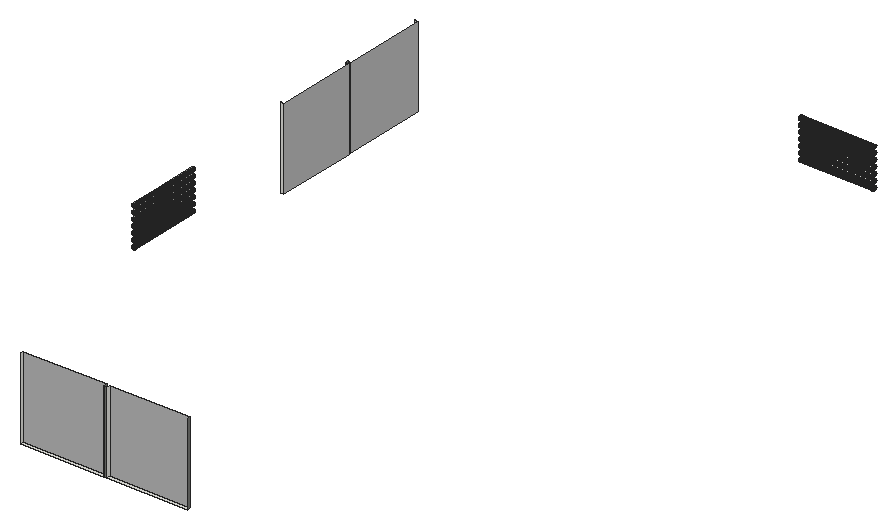
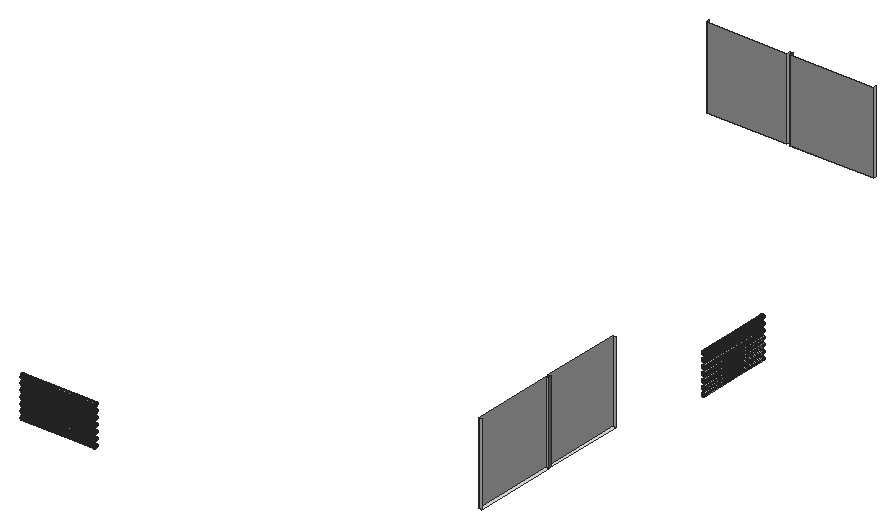
# SketchUp Ruby script. Lengths in inches.
U = 1.inch
M = Sketchup.active_model
def pt(a) = Geom::Point3d.new(a.map { |v| v * U })
def face(e, loops, mat)
  f = e.add_face(loops[0].map { |a| pt(a) })
  loops[1..].each { |l| e.add_face(l.map { |a| pt(a) }).erase! }
  f.material = f.back_material = mat if mat
  f
end
# faces: each face lists its corners as indices into pts; further lists are holes
def faces(e, pts, list, mat = nil) = list.each { |f| face(e, (f[0].is_a?(Array) ? f : [f]).map { |l| l.map { |i| pts[i] } }, mat) }
# xy, xz, yz: faces in a plane at the given z, y or x. An outline is a flat list of corners, or four numbers for a rectangle; further outlines are holes
def ring(l) = l.size == 4 ? [[l[0], l[1]], [l[2], l[1]], [l[2], l[3]], [l[0], l[3]]] : l.each_slice(2).to_a
def flat(e, list, mat, &to3) = list.each { |f| face(e, (f[0].is_a?(Array) ? f : [f]).map { |l| ring(l).map { |u, v| to3.(u, v) } }, mat) }
def xy(e, z, list, mat = nil) = flat(e, list, mat) { |x, y| [x, y, z] }
def xz(e, y, list, mat = nil) = flat(e, list, mat) { |x, z| [x, y, z] }
def yz(e, x, list, mat = nil) = flat(e, list, mat) { |y, z| [x, y, z] }
def lines(e, pts, list) = list.each { |a, b| e.add_line(pt(pts[a]), pt(pts[b])) }
# prism: a flat outline (further loops are holes) pulled along v
def prism(e, loops, v, mat = nil)
  f = face(e, loops, mat); d = Geom::Vector3d.new(v.map { |x| x * U })
  f.pushpull(f.normal.samedirection?(d) ? d.length : -d.length)
end
def box(e, o, s, mat = nil) = prism(e, [[o, [o[0] + s[0], o[1], o[2]], [o[0] + s[0], o[1] + s[1], o[2]], [o[0], o[1] + s[1], o[2]]]], [0, 0, s[2]], mat)
def at(x, y, z, deg = 0) = Geom::Transformation.translation(pt([x, y, z])) * Geom::Transformation.rotation(ORIGIN, Z_AXIS, deg.degrees)
def axes(o, x, y, z) = Geom::Transformation.new([*x, 0, *y, 0, *z, 0, *pt(o).to_a, 1])
def part(name) = M.definitions.add(name)
# library, detail: a bought-in or finely detailed component or shape, given as its bounding box
def library(name, o, s) = part(name).tap { |d| box(d.entities, o, s) }
def detail(e, o, s) = box(e.add_group.entities, o, s)
def put(e, d, t, mat = nil) = e.add_instance(d, t).tap { |i| i.material = mat if mat }
def group(e, t, mat = nil) = e.add_group.tap { |g| g.transformation = t; g.material = mat if mat }.entities
root = M.entities
M.materials.add("[Metal Seamed]").color = [118, 119, 115]
M.materials.add("[Mirror 01]").color = [185, 185, 185]
xy(root,539.76,[[312.65,102.8125,473.9375,108.8125],[479.9375,102.8125,635.22,108.8125],[138,949.59,144,1104.875],[138,1110.875,144,1272.16]])
xz(root,102.8125,[[473.9375,539.76,479.9375,696.625]],"[Metal Seamed]")
xz(root,108.8125,[[312.65,539.76,473.9375,696.625],[479.9375,539.76,635.22,696.625]],"[Mirror 01]")
xz(root,949.59,[[138,539.76,144,696.625]])
xz(root,1104.875,[[138,539.76,144,696.625]])
xz(root,1110.875,[[138,539.76,144,696.625]])
xz(root,1272.16,[[138,539.76,144,696.625]])
yz(root,138,[[1104.875,539.76,1110.875,696.625]],"[Metal Seamed]")
yz(root,144,[[949.59,539.76,1104.875,696.625],[1110.875,539.76,1272.16,696.625]],"[Mirror 01]")
yz(root,312.65,[[102.8125,539.76,108.8125,696.625]])
yz(root,473.9375,[[102.8125,539.76,108.8125,696.625]],"[Metal Seamed]")
yz(root,479.9375,[[102.8125,539.76,108.8125,696.625]])
yz(root,635.22,[[102.8125,539.76,108.8125,696.625]],"[Metal Seamed]")
p = [[83.53,662.8,549.02],[82.57,662.8,549.14],[82.57,806.17,549.14],[83.53,806.17,549.02],[84.48,662.8,549.14],[84.48,806.17,549.14],
  [697.99,1500.33,549.14],[697.99,1501.28,549.02],[841.36,1501.28,549.02],[841.36,1500.33,549.14],[697.99,1502.24,549.14],[841.36,1502.24,549.14],
  [81.68,662.8,549.51],[81.68,806.17,549.51],[85.37,662.8,549.51],[85.37,806.17,549.51],[697.99,1499.44,549.51],[841.36,1499.44,549.51],
  [697.99,1503.13,549.51],[841.36,1503.13,549.51],[80.92,662.8,550.1],[80.92,806.17,550.1],[86.13,662.8,550.1],[86.13,806.17,550.1],
  [697.99,1498.68,550.1],[841.36,1498.68,550.1],[697.99,1503.89,550.1],[841.36,1503.89,550.1],[80.33,662.8,550.86],[80.33,806.17,550.86],
  [86.72,662.8,550.86],[86.72,806.17,550.86],[697.99,1498.09,550.86],[841.36,1498.09,550.86],[697.99,1504.48,550.86],[841.36,1504.48,550.86],
  [79.97,662.8,551.75],[79.97,806.17,551.75],[87.09,662.8,551.75],[87.09,806.17,551.75],[697.99,1497.72,551.75],[841.36,1497.72,551.75],
  [697.99,1504.85,551.75],[841.36,1504.85,551.75],[79.84,662.8,552.7],[79.84,806.17,552.7],[87.21,662.8,552.7],[87.21,806.17,552.7],
  [697.99,1497.6,552.7],[841.36,1497.6,552.7],[697.99,1504.97,552.7],[841.36,1504.97,552.7],[79.97,662.8,553.66],[79.97,806.17,553.66],
  [87.09,662.8,553.66],[87.09,806.17,553.66],[697.99,1497.72,553.66],[841.36,1497.72,553.66],[697.99,1504.85,553.66],[841.36,1504.85,553.66],
  [80.33,662.8,554.55],[80.33,806.17,554.55],[86.72,662.8,554.55],[86.72,806.17,554.55],[697.99,1498.09,554.55],[841.36,1498.09,554.55],
  [697.99,1504.48,554.55],[841.36,1504.48,554.55],[80.92,662.8,555.3125],[80.92,806.17,555.3125],[86.13,662.8,555.3125],[86.13,806.17,555.3125],
  [697.99,1498.68,555.3125],[841.36,1498.68,555.3125],[697.99,1503.89,555.3125],[841.36,1503.89,555.3125],[81.68,662.8,555.9],[81.68,806.17,555.9],
  [85.37,662.8,555.9],[85.37,806.17,555.9],[697.99,1499.44,555.9],[841.36,1499.44,555.9],[697.99,1503.13,555.9],[841.36,1503.13,555.9],
  [82.57,662.8,556.27],[82.57,806.17,556.27],[84.48,662.8,556.27],[84.48,806.17,556.27],[697.99,1500.33,556.27],[841.36,1500.33,556.27],
  [697.99,1502.24,556.27],[841.36,1502.24,556.27],[83.53,662.8,556.39],[83.53,806.17,556.39],[697.99,1501.28,556.39],[841.36,1501.28,556.39],
  [83.53,662.8,561.02],[82.57,662.8,561.14],[82.57,806.17,561.14],[83.53,806.17,561.02],[84.48,662.8,561.14],[84.48,806.17,561.14],
  [697.99,1500.33,561.14],[697.99,1501.28,561.02],[841.36,1501.28,561.02],[841.36,1500.33,561.14],[697.99,1502.24,561.14],[841.36,1502.24,561.14],
  [81.68,662.8,561.51],[81.68,806.17,561.51],[85.37,662.8,561.51],[85.37,806.17,561.51],[697.99,1499.44,561.51],[841.36,1499.44,561.51],
  [697.99,1503.13,561.51],[841.36,1503.13,561.51],[80.92,662.8,562.1],[80.92,806.17,562.1],[86.13,662.8,562.1],[86.13,806.17,562.1],
  [697.99,1498.68,562.1],[841.36,1498.68,562.1],[697.99,1503.89,562.1],[841.36,1503.89,562.1],[80.33,662.8,562.86],[80.33,806.17,562.86],
  [86.72,662.8,562.86],[86.72,806.17,562.86],[697.99,1498.09,562.86],[841.36,1498.09,562.86],[697.99,1504.48,562.86],[841.36,1504.48,562.86],
  [79.97,662.8,563.75],[79.97,806.17,563.75],[87.09,662.8,563.75],[87.09,806.17,563.75],[697.99,1497.72,563.75],[841.36,1497.72,563.75],
  [697.99,1504.85,563.75],[841.36,1504.85,563.75],[79.84,662.8,564.7],[79.84,806.17,564.7],[87.21,662.8,564.7],[87.21,806.17,564.7],
  [697.99,1497.6,564.7],[841.36,1497.6,564.7],[697.99,1504.97,564.7],[841.36,1504.97,564.7],[79.97,662.8,565.66],[79.97,806.17,565.66],
  [87.09,662.8,565.66],[87.09,806.17,565.66],[697.99,1497.72,565.66],[841.36,1497.72,565.66],[697.99,1504.85,565.66],[841.36,1504.85,565.66],
  [80.33,662.8,566.55],[80.33,806.17,566.55],[86.72,662.8,566.55],[86.72,806.17,566.55],[697.99,1498.09,566.55],[841.36,1498.09,566.55],
  [697.99,1504.48,566.55],[841.36,1504.48,566.55],[80.92,662.8,567.3125],[80.92,806.17,567.3125],[86.13,662.8,567.3125],[86.13,806.17,567.3125],
  [697.99,1498.68,567.3125],[841.36,1498.68,567.3125],[697.99,1503.89,567.3125],[841.36,1503.89,567.3125],[81.68,662.8,567.9],[81.68,806.17,567.9],
  [85.37,662.8,567.9],[85.37,806.17,567.9],[697.99,1499.44,567.9],[841.36,1499.44,567.9],[697.99,1503.13,567.9],[841.36,1503.13,567.9],
  [82.57,662.8,568.27],[82.57,806.17,568.27],[84.48,662.8,568.27],[84.48,806.17,568.27],[697.99,1500.33,568.27],[841.36,1500.33,568.27],
  [697.99,1502.24,568.27],[841.36,1502.24,568.27],[83.53,662.8,568.39],[83.53,806.17,568.39],[697.99,1501.28,568.39],[841.36,1501.28,568.39],
  [83.53,662.8,573.02],[82.57,662.8,573.14],[82.57,806.17,573.14],[83.53,806.17,573.02],[84.48,662.8,573.14],[84.48,806.17,573.14],
  [697.99,1500.33,573.14],[697.99,1501.28,573.02],[841.36,1501.28,573.02],[841.36,1500.33,573.14],[697.99,1502.24,573.14],[841.36,1502.24,573.14],
  [81.68,662.8,573.51],[81.68,806.17,573.51],[85.37,662.8,573.51],[85.37,806.17,573.51],[697.99,1499.44,573.51],[841.36,1499.44,573.51],
  [697.99,1503.13,573.51],[841.36,1503.13,573.51],[80.92,662.8,574.1],[80.92,806.17,574.1],[86.13,662.8,574.1],[86.13,806.17,574.1],
  [697.99,1498.68,574.1],[841.36,1498.68,574.1],[697.99,1503.89,574.1],[841.36,1503.89,574.1],[80.33,662.8,574.86],[80.33,806.17,574.86],
  [86.72,662.8,574.86],[86.72,806.17,574.86],[697.99,1498.09,574.86],[841.36,1498.09,574.86],[697.99,1504.48,574.86],[841.36,1504.48,574.86],
  [79.97,662.8,575.75],[79.97,806.17,575.75],[87.09,662.8,575.75],[87.09,806.17,575.75],[697.99,1497.72,575.75],[841.36,1497.72,575.75],
  [697.99,1504.85,575.75],[841.36,1504.85,575.75],[79.84,662.8,576.7],[79.84,806.17,576.7],[87.21,662.8,576.7],[87.21,806.17,576.7],
  [697.99,1497.6,576.7],[841.36,1497.6,576.7],[697.99,1504.97,576.7],[841.36,1504.97,576.7],[79.97,662.8,577.66],[79.97,806.17,577.66],
  [87.09,662.8,577.66],[87.09,806.17,577.66],[697.99,1497.72,577.66],[841.36,1497.72,577.66],[697.99,1504.85,577.66],[841.36,1504.85,577.66],
  [80.33,662.8,578.55],[80.33,806.17,578.55],[86.72,662.8,578.55],[86.72,806.17,578.55],[697.99,1498.09,578.55],[841.36,1498.09,578.55],
  [697.99,1504.48,578.55],[841.36,1504.48,578.55],[80.92,662.8,579.3125],[80.92,806.17,579.3125],[86.13,662.8,579.3125],[86.13,806.17,579.3125],
  [697.99,1498.68,579.3125],[841.36,1498.68,579.3125],[697.99,1503.89,579.3125],[841.36,1503.89,579.3125],[81.68,662.8,579.9],[81.68,806.17,579.9],
  [85.37,662.8,579.9],[85.37,806.17,579.9],[697.99,1499.44,579.9],[841.36,1499.44,579.9],[697.99,1503.13,579.9],[841.36,1503.13,579.9],
  [82.57,662.8,580.27],[82.57,806.17,580.27],[84.48,662.8,580.27],[84.48,806.17,580.27],[697.99,1500.33,580.27],[841.36,1500.33,580.27],
  [697.99,1502.24,580.27],[841.36,1502.24,580.27],[83.53,662.8,580.39],[83.53,806.17,580.39],[697.99,1501.28,580.39],[841.36,1501.28,580.39],
  [83.53,662.8,585.02],[82.57,662.8,585.14],[82.57,806.17,585.14],[83.53,806.17,585.02],[84.48,662.8,585.14],[84.48,806.17,585.14],
  [697.99,1500.33,585.14],[697.99,1501.28,585.02],[841.36,1501.28,585.02],[841.36,1500.33,585.14],[697.99,1502.24,585.14],[841.36,1502.24,585.14],
  [81.68,662.8,585.51],[81.68,806.17,585.51],[85.37,662.8,585.51],[85.37,806.17,585.51],[697.99,1499.44,585.51],[841.36,1499.44,585.51],
  [697.99,1503.13,585.51],[841.36,1503.13,585.51],[80.92,662.8,586.1],[80.92,806.17,586.1],[86.13,662.8,586.1],[86.13,806.17,586.1],
  [697.99,1498.68,586.1],[841.36,1498.68,586.1],[697.99,1503.89,586.1],[841.36,1503.89,586.1],[80.33,662.8,586.86],[80.33,806.17,586.86],
  [86.72,662.8,586.86],[86.72,806.17,586.86],[697.99,1498.09,586.86],[841.36,1498.09,586.86],[697.99,1504.48,586.86],[841.36,1504.48,586.86],
  [79.97,662.8,587.75],[79.97,806.17,587.75],[87.09,662.8,587.75],[87.09,806.17,587.75],[697.99,1497.72,587.75],[841.36,1497.72,587.75],
  [697.99,1504.85,587.75],[841.36,1504.85,587.75],[79.84,662.8,588.7],[79.84,806.17,588.7],[87.21,662.8,588.7],[87.21,806.17,588.7],
  [697.99,1497.6,588.7],[841.36,1497.6,588.7],[697.99,1504.97,588.7],[841.36,1504.97,588.7],[79.97,662.8,589.66],[79.97,806.17,589.66],
  [87.09,662.8,589.66],[87.09,806.17,589.66],[697.99,1497.72,589.66],[841.36,1497.72,589.66],[697.99,1504.85,589.66],[841.36,1504.85,589.66],
  [80.33,662.8,590.55],[80.33,806.17,590.55],[86.72,662.8,590.55],[86.72,806.17,590.55],[697.99,1498.09,590.55],[841.36,1498.09,590.55],
  [697.99,1504.48,590.55],[841.36,1504.48,590.55],[80.92,662.8,591.3125],[80.92,806.17,591.3125],[86.13,662.8,591.3125],[86.13,806.17,591.3125],
  [697.99,1498.68,591.3125],[841.36,1498.68,591.3125],[697.99,1503.89,591.3125],[841.36,1503.89,591.3125],[81.68,662.8,591.9],[81.68,806.17,591.9],
  [85.37,662.8,591.9],[85.37,806.17,591.9],[697.99,1499.44,591.9],[841.36,1499.44,591.9],[697.99,1503.13,591.9],[841.36,1503.13,591.9],
  [82.57,662.8,592.27],[82.57,806.17,592.27],[84.48,662.8,592.27],[84.48,806.17,592.27],[697.99,1500.33,592.27],[841.36,1500.33,592.27],
  [697.99,1502.24,592.27],[841.36,1502.24,592.27],[83.53,662.8,592.39],[83.53,806.17,592.39],[697.99,1501.28,592.39],[841.36,1501.28,592.39],
  [83.53,662.8,597.02],[82.57,662.8,597.14],[82.57,806.17,597.14],[83.53,806.17,597.02],[84.48,662.8,597.14],[84.48,806.17,597.14],
  [697.99,1500.33,597.14],[697.99,1501.28,597.02],[841.36,1501.28,597.02],[841.36,1500.33,597.14],[697.99,1502.24,597.14],[841.36,1502.24,597.14],
  [81.68,662.8,597.51],[81.68,806.17,597.51],[85.37,662.8,597.51],[85.37,806.17,597.51],[697.99,1499.44,597.51],[841.36,1499.44,597.51],
  [697.99,1503.13,597.51],[841.36,1503.13,597.51],[80.92,662.8,598.1],[80.92,806.17,598.1],[86.13,662.8,598.1],[86.13,806.17,598.1],
  [697.99,1498.68,598.1],[841.36,1498.68,598.1],[697.99,1503.89,598.1],[841.36,1503.89,598.1],[80.33,662.8,598.86],[80.33,806.17,598.86],
  [86.72,662.8,598.86],[86.72,806.17,598.86],[697.99,1498.09,598.86],[841.36,1498.09,598.86],[697.99,1504.48,598.86],[841.36,1504.48,598.86],
  [79.97,662.8,599.75],[79.97,806.17,599.75],[87.09,662.8,599.75],[87.09,806.17,599.75],[697.99,1497.72,599.75],[841.36,1497.72,599.75],
  [697.99,1504.85,599.75],[841.36,1504.85,599.75],[79.84,662.8,600.7],[79.84,806.17,600.7],[87.21,662.8,600.7],[87.21,806.17,600.7],
  [697.99,1497.6,600.7],[841.36,1497.6,600.7],[697.99,1504.97,600.7],[841.36,1504.97,600.7],[79.97,662.8,601.66],[79.97,806.17,601.66],
  [87.09,662.8,601.66],[87.09,806.17,601.66],[697.99,1497.72,601.66],[841.36,1497.72,601.66],[697.99,1504.85,601.66],[841.36,1504.85,601.66],
  [80.33,662.8,602.55],[80.33,806.17,602.55],[86.72,662.8,602.55],[86.72,806.17,602.55],[697.99,1498.09,602.55],[841.36,1498.09,602.55],
  [697.99,1504.48,602.55],[841.36,1504.48,602.55],[80.92,662.8,603.3125],[80.92,806.17,603.3125],[86.13,662.8,603.3125],[86.13,806.17,603.3125],
  [697.99,1498.68,603.3125],[841.36,1498.68,603.3125],[697.99,1503.89,603.3125],[841.36,1503.89,603.3125],[81.68,662.8,603.9],[81.68,806.17,603.9],
  [85.37,662.8,603.9],[85.37,806.17,603.9],[697.99,1499.44,603.9],[841.36,1499.44,603.9],[697.99,1503.13,603.9],[841.36,1503.13,603.9],
  [82.57,662.8,604.27],[82.57,806.17,604.27],[84.48,662.8,604.27],[84.48,806.17,604.27],[697.99,1500.33,604.27],[841.36,1500.33,604.27],
  [697.99,1502.24,604.27],[841.36,1502.24,604.27],[83.53,662.8,604.39],[83.53,806.17,604.39],[697.99,1501.28,604.39],[841.36,1501.28,604.39],
  [83.53,662.8,609.02],[82.57,662.8,609.14],[82.57,806.17,609.14],[83.53,806.17,609.02],[84.48,662.8,609.14],[84.48,806.17,609.14],
  [697.99,1500.33,609.14],[697.99,1501.28,609.02],[841.36,1501.28,609.02],[841.36,1500.33,609.14],[697.99,1502.24,609.14],[841.36,1502.24,609.14],
  [81.68,662.8,609.51],[81.68,806.17,609.51],[85.37,662.8,609.51],[85.37,806.17,609.51],[697.99,1499.44,609.51],[841.36,1499.44,609.51],
  [697.99,1503.13,609.51],[841.36,1503.13,609.51],[80.92,662.8,610.1],[80.92,806.17,610.1],[86.13,662.8,610.1],[86.13,806.17,610.1],
  [697.99,1498.68,610.1],[841.36,1498.68,610.1],[697.99,1503.89,610.1],[841.36,1503.89,610.1],[80.33,662.8,610.86],[80.33,806.17,610.86],
  [86.72,662.8,610.86],[86.72,806.17,610.86],[697.99,1498.09,610.86],[841.36,1498.09,610.86],[697.99,1504.48,610.86],[841.36,1504.48,610.86],
  [79.97,662.8,611.75],[79.97,806.17,611.75],[87.09,662.8,611.75],[87.09,806.17,611.75],[697.99,1497.72,611.75],[841.36,1497.72,611.75],
  [697.99,1504.85,611.75],[841.36,1504.85,611.75],[79.84,662.8,612.7],[79.84,806.17,612.7],[87.21,662.8,612.7],[87.21,806.17,612.7],
  [697.99,1497.6,612.7],[841.36,1497.6,612.7],[697.99,1504.97,612.7],[841.36,1504.97,612.7],[79.97,662.8,613.66],[79.97,806.17,613.66],
  [87.09,662.8,613.66],[87.09,806.17,613.66],[697.99,1497.72,613.66],[841.36,1497.72,613.66],[697.99,1504.85,613.66],[841.36,1504.85,613.66],
  [80.33,662.8,614.55],[80.33,806.17,614.55],[86.72,662.8,614.55],[86.72,806.17,614.55],[697.99,1498.09,614.55],[841.36,1498.09,614.55],
  [697.99,1504.48,614.55],[841.36,1504.48,614.55],[80.92,662.8,615.3125],[80.92,806.17,615.3125],[86.13,662.8,615.3125],[86.13,806.17,615.3125],
  [697.99,1498.68,615.3125],[841.36,1498.68,615.3125],[697.99,1503.89,615.3125],[841.36,1503.89,615.3125],[81.68,662.8,615.9],[81.68,806.17,615.9],
  [85.37,662.8,615.9],[85.37,806.17,615.9],[697.99,1499.44,615.9],[841.36,1499.44,615.9],[697.99,1503.13,615.9],[841.36,1503.13,615.9],
  [82.57,662.8,616.27],[82.57,806.17,616.27],[84.48,662.8,616.27],[84.48,806.17,616.27],[697.99,1500.33,616.27],[841.36,1500.33,616.27],
  [697.99,1502.24,616.27],[841.36,1502.24,616.27],[83.53,662.8,616.39],[83.53,806.17,616.39],[697.99,1501.28,616.39],[841.36,1501.28,616.39],
  [83.53,662.8,621.02],[82.57,662.8,621.14],[82.57,806.17,621.14],[83.53,806.17,621.02],[84.48,662.8,621.14],[84.48,806.17,621.14],
  [697.99,1500.33,621.14],[697.99,1501.28,621.02],[841.36,1501.28,621.02],[841.36,1500.33,621.14],[697.99,1502.24,621.14],[841.36,1502.24,621.14],
  [81.68,662.8,621.51],[81.68,806.17,621.51],[85.37,662.8,621.51],[85.37,806.17,621.51],[697.99,1499.44,621.51],[841.36,1499.44,621.51],
  [697.99,1503.13,621.51],[841.36,1503.13,621.51],[80.92,662.8,622.1],[80.92,806.17,622.1],[86.13,662.8,622.1],[86.13,806.17,622.1],
  [697.99,1498.68,622.1],[841.36,1498.68,622.1],[697.99,1503.89,622.1],[841.36,1503.89,622.1],[80.33,662.8,622.86],[80.33,806.17,622.86],
  [86.72,662.8,622.86],[86.72,806.17,622.86],[697.99,1498.09,622.86],[841.36,1498.09,622.86],[697.99,1504.48,622.86],[841.36,1504.48,622.86],
  [79.97,662.8,623.75],[79.97,806.17,623.75],[87.09,662.8,623.75],[87.09,806.17,623.75],[697.99,1497.72,623.75],[841.36,1497.72,623.75],
  [697.99,1504.85,623.75],[841.36,1504.85,623.75],[79.84,662.8,624.7],[79.84,806.17,624.7],[87.21,662.8,624.7],[87.21,806.17,624.7],
  [697.99,1497.6,624.7],[841.36,1497.6,624.7],[697.99,1504.97,624.7],[841.36,1504.97,624.7],[79.97,662.8,625.66],[79.97,806.17,625.66],
  [87.09,662.8,625.66],[87.09,806.17,625.66],[697.99,1497.72,625.66],[841.36,1497.72,625.66],[697.99,1504.85,625.66],[841.36,1504.85,625.66],
  [80.33,662.8,626.55],[80.33,806.17,626.55],[86.72,662.8,626.55],[86.72,806.17,626.55],[697.99,1498.09,626.55],[841.36,1498.09,626.55],
  [697.99,1504.48,626.55],[841.36,1504.48,626.55],[80.92,662.8,627.3125],[80.92,806.17,627.3125],[86.13,662.8,627.3125],[86.13,806.17,627.3125],
  [697.99,1498.68,627.3125],[841.36,1498.68,627.3125],[697.99,1503.89,627.3125],[841.36,1503.89,627.3125],[81.68,662.8,627.9],[81.68,806.17,627.9],
  [85.37,662.8,627.9],[85.37,806.17,627.9],[697.99,1499.44,627.9],[841.36,1499.44,627.9],[697.99,1503.13,627.9],[841.36,1503.13,627.9],
  [82.57,662.8,628.27],[82.57,806.17,628.27],[84.48,662.8,628.27],[84.48,806.17,628.27],[697.99,1500.33,628.27],[841.36,1500.33,628.27],
  [697.99,1502.24,628.27],[841.36,1502.24,628.27],[83.53,662.8,628.39],[83.53,806.17,628.39],[697.99,1501.28,628.39],[841.36,1501.28,628.39]]
faces(root,p,[[0,1,2,3],[4,0,3,5],[6,7,8,9],[7,10,11,8],[1,12,13,2],[14,4,5,15],[16,6,9,17],[10,18,19,11],
  [12,20,21,13],[22,14,15,23],[24,16,17,25],[18,26,27,19],[20,28,29,21],[30,22,23,31],[32,24,25,33],[26,34,35,27],
  [28,36,37,29],[38,30,31,39],[40,32,33,41],[34,42,43,35],[36,44,45,37],[46,38,39,47],[48,40,41,49],[42,50,51,43],
  [44,52,53,45],[54,46,47,55],[56,48,49,57],[50,58,59,51],[52,60,61,53],[62,54,55,63],[64,56,57,65],[58,66,67,59],
  [60,68,69,61],[70,62,63,71],[72,64,65,73],[66,74,75,67],[68,76,77,69],[78,70,71,79],[80,72,73,81],[74,82,83,75],
  [76,84,85,77],[86,78,79,87],[88,80,81,89],[82,90,91,83],[84,92,93,85],[92,86,87,93],[94,88,89,95],[90,94,95,91],
  [96,97,98,99],[100,96,99,101],[102,103,104,105],[103,106,107,104],[97,108,109,98],[110,100,101,111],[112,102,105,113],[106,114,115,107],
  [108,116,117,109],[118,110,111,119],[120,112,113,121],[114,122,123,115],[116,124,125,117],[126,118,119,127],[128,120,121,129],[122,130,131,123],
  [124,132,133,125],[134,126,127,135],[136,128,129,137],[130,138,139,131],[132,140,141,133],[142,134,135,143],[144,136,137,145],[138,146,147,139],
  [140,148,149,141],[150,142,143,151],[152,144,145,153],[146,154,155,147],[148,156,157,149],[158,150,151,159],[160,152,153,161],[154,162,163,155],
  [156,164,165,157],[166,158,159,167],[168,160,161,169],[162,170,171,163],[164,172,173,165],[174,166,167,175],[176,168,169,177],[170,178,179,171],
  [172,180,181,173],[182,174,175,183],[184,176,177,185],[178,186,187,179],[180,188,189,181],[188,182,183,189],[190,184,185,191],[186,190,191,187],
  [192,193,194,195],[196,192,195,197],[198,199,200,201],[199,202,203,200],[193,204,205,194],[206,196,197,207],[208,198,201,209],[202,210,211,203],
  [204,212,213,205],[214,206,207,215],[216,208,209,217],[210,218,219,211],[212,220,221,213],[222,214,215,223],[224,216,217,225],[218,226,227,219],
  [220,228,229,221],[230,222,223,231],[232,224,225,233],[226,234,235,227],[228,236,237,229],[238,230,231,239],[240,232,233,241],[234,242,243,235],
  [236,244,245,237],[246,238,239,247],[248,240,241,249],[242,250,251,243],[244,252,253,245],[254,246,247,255],[256,248,249,257],[250,258,259,251],
  [252,260,261,253],[262,254,255,263],[264,256,257,265],[258,266,267,259],[260,268,269,261],[270,262,263,271],[272,264,265,273],[266,274,275,267],
  [268,276,277,269],[278,270,271,279],[280,272,273,281],[274,282,283,275],[276,284,285,277],[284,278,279,285],[286,280,281,287],[282,286,287,283],
  [288,289,290,291],[292,288,291,293],[294,295,296,297],[295,298,299,296],[289,300,301,290],[302,292,293,303],[304,294,297,305],[298,306,307,299],
  [300,308,309,301],[310,302,303,311],[312,304,305,313],[306,314,315,307],[308,316,317,309],[318,310,311,319],[320,312,313,321],[314,322,323,315],
  [316,324,325,317],[326,318,319,327],[328,320,321,329],[322,330,331,323],[324,332,333,325],[334,326,327,335],[336,328,329,337],[330,338,339,331],
  [332,340,341,333],[342,334,335,343],[344,336,337,345],[338,346,347,339],[340,348,349,341],[350,342,343,351],[352,344,345,353],[346,354,355,347],
  [348,356,357,349],[358,350,351,359],[360,352,353,361],[354,362,363,355],[356,364,365,357],[366,358,359,367],[368,360,361,369],[362,370,371,363],
  [364,372,373,365],[374,366,367,375],[376,368,369,377],[370,378,379,371],[372,380,381,373],[380,374,375,381],[382,376,377,383],[378,382,383,379],
  [384,385,386,387],[388,384,387,389],[390,391,392,393],[391,394,395,392],[385,396,397,386],[398,388,389,399],[400,390,393,401],[394,402,403,395],
  [396,404,405,397],[406,398,399,407],[408,400,401,409],[402,410,411,403],[404,412,413,405],[414,406,407,415],[416,408,409,417],[410,418,419,411],
  [412,420,421,413],[422,414,415,423],[424,416,417,425],[418,426,427,419],[420,428,429,421],[430,422,423,431],[432,424,425,433],[426,434,435,427],
  [428,436,437,429],[438,430,431,439],[440,432,433,441],[434,442,443,435],[436,444,445,437],[446,438,439,447],[448,440,441,449],[442,450,451,443],
  [444,452,453,445],[454,446,447,455],[456,448,449,457],[450,458,459,451],[452,460,461,453],[462,454,455,463],[464,456,457,465],[458,466,467,459],
  [460,468,469,461],[470,462,463,471],[472,464,465,473],[466,474,475,467],[468,476,477,469],[476,470,471,477],[478,472,473,479],[474,478,479,475],
  [480,481,482,483],[484,480,483,485],[486,487,488,489],[487,490,491,488],[481,492,493,482],[494,484,485,495],[496,486,489,497],[490,498,499,491],
  [492,500,501,493],[502,494,495,503],[504,496,497,505],[498,506,507,499],[500,508,509,501],[510,502,503,511],[512,504,505,513],[506,514,515,507],
  [508,516,517,509],[518,510,511,519],[520,512,513,521],[514,522,523,515],[516,524,525,517],[526,518,519,527],[528,520,521,529],[522,530,531,523],
  [524,532,533,525],[534,526,527,535],[536,528,529,537],[530,538,539,531],[532,540,541,533],[542,534,535,543],[544,536,537,545],[538,546,547,539],
  [540,548,549,541],[550,542,543,551],[552,544,545,553],[546,554,555,547],[548,556,557,549],[558,550,551,559],[560,552,553,561],[554,562,563,555],
  [556,564,565,557],[566,558,559,567],[568,560,561,569],[562,570,571,563],[564,572,573,565],[572,566,567,573],[574,568,569,575],[570,574,575,571],
  [576,577,578,579],[580,576,579,581],[582,583,584,585],[583,586,587,584],[577,588,589,578],[590,580,581,591],[592,582,585,593],[586,594,595,587],
  [588,596,597,589],[598,590,591,599],[600,592,593,601],[594,602,603,595],[596,604,605,597],[606,598,599,607],[608,600,601,609],[602,610,611,603],
  [604,612,613,605],[614,606,607,615],[616,608,609,617],[610,618,619,611],[612,620,621,613],[622,614,615,623],[624,616,617,625],[618,626,627,619],
  [620,628,629,621],[630,622,623,631],[632,624,625,633],[626,634,635,627],[628,636,637,629],[638,630,631,639],[640,632,633,641],[634,642,643,635],
  [636,644,645,637],[646,638,639,647],[648,640,641,649],[642,650,651,643],[644,652,653,645],[654,646,647,655],[656,648,649,657],[650,658,659,651],
  [652,660,661,653],[662,654,655,663],[664,656,657,665],[658,666,667,659],[660,668,669,661],[668,662,663,669],[670,664,665,671],[666,670,671,667]])
